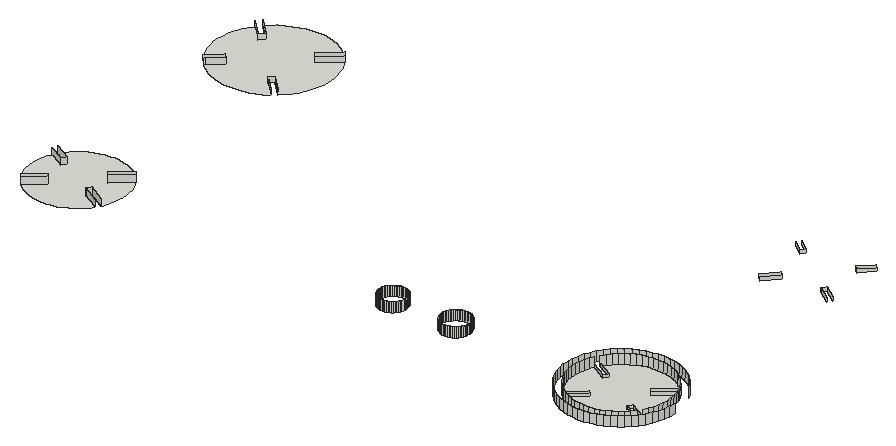
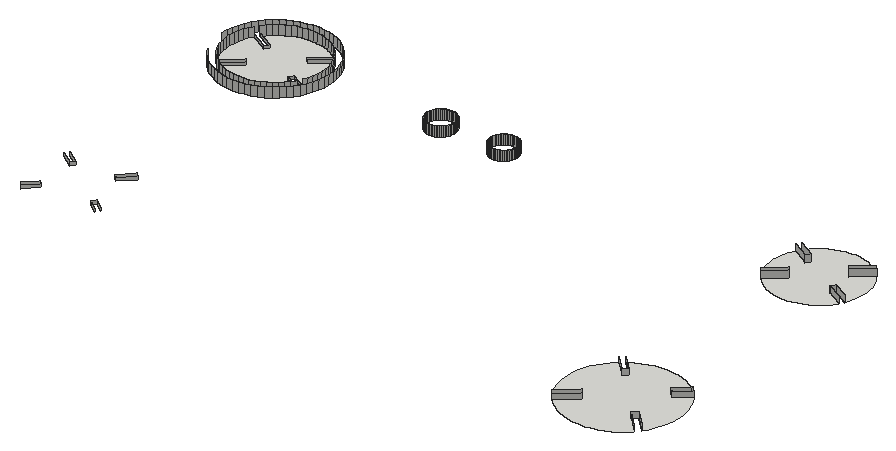
# SketchUp Ruby script. Lengths in inches.
U = 1.inch
M = Sketchup.active_model
def pt(a) = Geom::Point3d.new(a.map { |v| v * U })
def face(e, loops, mat)
  f = e.add_face(loops[0].map { |a| pt(a) })
  loops[1..].each { |l| e.add_face(l.map { |a| pt(a) }).erase! }
  f.material = f.back_material = mat if mat
  f
end
# faces: each face lists its corners as indices into pts; further lists are holes
def faces(e, pts, list, mat = nil) = list.each { |f| face(e, (f[0].is_a?(Array) ? f : [f]).map { |l| l.map { |i| pts[i] } }, mat) }
# xy, xz, yz: faces in a plane at the given z, y or x. An outline is a flat list of corners, or four numbers for a rectangle; further outlines are holes
def ring(l) = l.size == 4 ? [[l[0], l[1]], [l[2], l[1]], [l[2], l[3]], [l[0], l[3]]] : l.each_slice(2).to_a
def flat(e, list, mat, &to3) = list.each { |f| face(e, (f[0].is_a?(Array) ? f : [f]).map { |l| ring(l).map { |u, v| to3.(u, v) } }, mat) }
def xy(e, z, list, mat = nil) = flat(e, list, mat) { |x, y| [x, y, z] }
def xz(e, y, list, mat = nil) = flat(e, list, mat) { |x, z| [x, y, z] }
def yz(e, x, list, mat = nil) = flat(e, list, mat) { |y, z| [x, y, z] }
def lines(e, pts, list) = list.each { |a, b| e.add_line(pt(pts[a]), pt(pts[b])) }
# prism: a flat outline (further loops are holes) pulled along v
def prism(e, loops, v, mat = nil)
  f = face(e, loops, mat); d = Geom::Vector3d.new(v.map { |x| x * U })
  f.pushpull(f.normal.samedirection?(d) ? d.length : -d.length)
end
def box(e, o, s, mat = nil) = prism(e, [[o, [o[0] + s[0], o[1], o[2]], [o[0] + s[0], o[1] + s[1], o[2]], [o[0], o[1] + s[1], o[2]]]], [0, 0, s[2]], mat)
def at(x, y, z, deg = 0) = Geom::Transformation.translation(pt([x, y, z])) * Geom::Transformation.rotation(ORIGIN, Z_AXIS, deg.degrees)
def axes(o, x, y, z) = Geom::Transformation.new([*x, 0, *y, 0, *z, 0, *pt(o).to_a, 1])
def part(name) = M.definitions.add(name)
# library, detail: a bought-in or finely detailed component or shape, given as its bounding box
def library(name, o, s) = part(name).tap { |d| box(d.entities, o, s) }
def detail(e, o, s) = box(e.add_group.entities, o, s)
def put(e, d, t, mat = nil) = e.add_instance(d, t).tap { |i| i.material = mat if mat }
def group(e, t, mat = nil) = e.add_group.tap { |g| g.transformation = t; g.material = mat if mat }.entities
root = M.entities
xy(root,253.1875,[[844.95,632.14,846.82,632.24,848.68,632.53,850.49,633.01,852.24,633.6875,853.91,634.54,855.49,635.56,856.94,636.74,858.27,638.07,859.45,639.53,852.51,643.53,853.45,645.15,860.47,641.1,861.32,642.77,862,644.52,862.48,646.33,862.77,648.1875,862.875,650.06,862.77,651.93,862.48,653.79,862,655.6,861.32,657.35,860.47,659.02,859.45,660.59,852.77,654.76,851.61,656.05,858.27,662.05,856.94,663.38,855.49,664.56,853.91,665.58,852.24,666.43,850.49,667.1,848.68,667.59,846.82,667.88,844.95,667.98,843.08,667.88,841.23,667.59,839.41,667.1,837.66,666.43,835.99,665.58,834.42,664.56,832.96,663.38,831.63,662.05,830.45,660.59,829.43,659.02,835.82,655.33,834.88,653.71,828.58,657.35,827.91,655.6,827.42,653.79,827.13,651.93,827.03,650.06,827.13,648.1875,827.42,646.33,827.91,644.52,828.58,642.77,829.43,641.1,830.45,639.53,831.63,638.07,837.78,643.6,838.75,642.52,832.58,637.12,832.96,636.74,834.42,635.56,835.99,634.54,837.66,633.6875,839.41,633.01,841.23,632.53,843.08,632.24],[634.4375,632.64,636.26,632.71,638.07,632.96,639.84,633.41,641.55,634.04,643.19,634.84,644.73,635.81,646.16,636.93,647.47,638.2,648.64,639.6,649.15,640.36,642.53,644.09,643.42,645.67,650.09,641.92,650.51,642.73,651.19,644.42,651.69,646.17,652.01,647.97,652.13,649.79,652.0625,651.61,651.8,653.42,651.36,655.18,650.73,656.9,649.93,658.53,648.96,660.08,642.65,654.57,641.46,655.95,647.84,661.51,646.57,662.82,645.17,663.99,643.65,665.01,642.04,665.86,640.35,666.54,638.6,667.04,636.8,667.35,634.98,667.48,633.16,667.41,631.35,667.15,629.58,666.71,627.87,666.08,626.23,665.28,624.69,664.31,623.25,663.19,621.95,661.92,620.78,660.52,619.76,659,625.78,655.61,624.89,654.02,618.91,657.39,618.23,655.7,617.73,653.95,617.41,652.15,617.29,650.33,617.36,648.51,617.61,646.7,618.06,644.93,618.6875,643.22,619.49,641.58,620.46,640.04,621.58,638.6,627.88,644.1,629.08,642.73,622.85,637.29,624.25,636.125,625.77,635.11,627.38,634.26,629.07,633.58,630.82,633.08,632.62,632.76],[634.71,723.48,636.95,723.59,639.16,723.94,641.33,724.53,643.42,725.33,645.42,726.35,647.3,727.57,641.99,732.875,643.57,734.45,649.04,728.98,650.63,730.5625,652.04,732.31,653.26,734.1875,654.28,736.19,655.08,738.28,655.66,740.44,656.01,742.66,656.13,744.9,656.01,747.14,655.66,749.35,655.08,751.52,654.28,753.61,653.26,755.61,652.04,757.49,645.15,751.5625,643.67,753.28,650.63,759.23,649.04,760.82,647.3,762.23,645.42,763.45,643.42,764.47,641.33,765.27,639.16,765.85,636.95,766.2,634.71,766.32,632.47,766.2,630.26,765.85,628.09,765.27,626,764.47,624,763.45,622.12,762.23,620.375,760.82,618.79,759.23,624.74,753.28,623.16,751.71,617.38,757.49,616.16,755.61,615.14,753.61,614.34,751.52,613.76,749.35,613.41,747.14,613.29,744.9,613.41,742.66,613.76,740.44,614.34,738.28,615.14,736.19,616.16,734.1875,617.38,732.31,618.09,731.4375,623.16,735.77,624.69,733.98,619.86,729.83,619.69,729.66,620.375,728.98,622.12,727.57,624,726.35,626,725.33,628.09,724.53,630.26,723.94,632.47,723.59]])
p = [[842.78,629.42,253.1875],[844.95,629.31,253.1875],[844.95,629.31,256.875],[842.78,629.42,256.875],[847.12,629.42,253.1875],[847.12,629.42,256.875],
  [840.64,629.76,253.1875],[840.64,629.76,256.875],[849.27,629.76,253.1875],[849.27,629.76,256.875],[838.54,630.32,253.1875],[838.54,630.32,256.875],
  [851.36,630.32,253.1875],[851.36,630.32,256.875],[836.51,631.1,253.1875],[836.51,631.1,256.875],[853.39,631.1,253.1875],[853.39,631.1,256.875],
  [834.58,632.09,253.1875],[834.58,632.09,256.875],[855.33,632.09,253.1875],[855.33,632.09,256.875],[832.76,633.27,253.1875],[832.76,633.27,256.875],
  [844.95,632.14,253.1875],[843.08,632.24,253.1875],[843.08,632.24,256.875],[844.95,632.14,256.875],[846.82,632.24,253.1875],[846.82,632.24,256.875],
  [857.15,633.27,253.1875],[857.15,633.27,256.875],[841.23,632.53,253.1875],[841.23,632.53,256.875],[848.68,632.53,253.1875],[848.68,632.53,256.875],
  [839.41,633.01,253.1875],[839.41,633.01,256.875],[850.49,633.01,253.1875],[850.49,633.01,256.875],[837.66,633.6875,253.1875],[837.66,633.6875,256.875],
  [852.24,633.6875,253.1875],[852.24,633.6875,256.875],[831.07,634.64,253.1875],[831.07,634.64,256.875],[858.84,634.64,253.1875],[858.84,634.64,256.875],
  [835.99,634.54,253.1875],[835.99,634.54,256.875],[853.91,634.54,253.1875],[853.91,634.54,256.875],[834.42,635.56,253.1875],[834.42,635.56,256.875],
  [855.49,635.56,253.1875],[855.49,635.56,256.875],[829.53,636.17,253.1875],[829.53,636.17,256.875],[860.37,636.17,253.1875],[860.37,636.17,256.875],
  [832.96,636.74,253.1875],[832.96,636.74,256.875],[856.94,636.74,253.1875],[856.94,636.74,256.875],[828.16,637.86,253.1875],[828.16,637.86,256.875],
  [861.74,637.86,253.1875],[861.74,637.86,256.875],[832.58,637.12,253.1875],[832.58,637.12,254.3125],[831.63,638.07,254.3125],[831.63,638.07,256.875],
  [858.27,638.07,253.1875],[858.27,638.07,256.875],[838.75,642.52,253.1875],[838.75,642.52,254.3125],[622.85,637.29,253.1875],[629.08,642.73,253.1875],
  [629.08,642.73,255.75],[622.85,637.29,255.75],[826.98,639.68,253.1875],[826.98,639.68,256.875],[862.92,639.68,253.1875],[862.92,639.68,256.875],
  [831.63,638.07,253.1875],[830.45,639.53,253.1875],[830.45,639.53,256.875],[837.78,643.6,253.1875],[837.78,643.6,254.3125],[859.45,639.53,253.1875],
  [859.45,639.53,256.875],[859.45,639.53,254.3125],[627.88,644.1,253.1875],[621.58,638.6,253.1875],[621.58,638.6,255.75],[627.88,644.1,255.75],
  [829.43,641.1,253.1875],[829.43,641.1,256.875],[852.51,643.53,253.1875],[852.51,643.53,254.3125],[826,641.62,253.1875],[826,641.62,256.875],
  [863.91,641.62,253.1875],[863.91,641.62,256.875],[642.53,644.09,253.1875],[649.15,640.36,253.1875],[649.15,640.36,255.75],[642.53,644.09,255.75],
  [828.58,642.77,253.1875],[828.58,642.77,256.875],[860.47,641.1,253.1875],[853.45,645.15,253.1875],[853.45,645.15,254.3125],[860.47,641.1,254.3125],
  [861.32,642.77,253.1875],[860.47,641.1,256.875],[861.32,642.77,256.875],[825.22,643.65,253.1875],[825.22,643.65,256.875],[864.6875,643.65,253.1875],
  [864.6875,643.65,256.875],[650.09,641.92,253.1875],[643.42,645.67,253.1875],[643.42,645.67,255.75],[650.09,641.92,255.75],[827.91,644.52,253.1875],
  [827.91,644.52,256.875],[862,644.52,253.1875],[862,644.52,256.875],[824.66,645.74,253.1875],[824.66,645.74,256.875],[865.25,645.74,253.1875],
  [865.25,645.74,256.875],[780.65,644.47,253.1875],[781.2,644.44,253.1875],[781.2,644.44,256.875],[780.65,644.47,256.875],[781.76,644.47,253.1875],
  [781.76,644.47,256.875],[780.1,644.56,253.1875],[780.1,644.56,256.875],[782.31,644.56,253.1875],[782.31,644.56,256.875],[827.42,646.33,253.1875],
  [827.42,646.33,256.875],[862.48,646.33,253.1875],[862.48,646.33,256.875],[779.5625,644.7,253.1875],[779.5625,644.7,256.875],[782.85,644.7,253.1875],
  [782.85,644.7,256.875],[755.79,644.8,253.1875],[756.3125,644.72,253.1875],[756.3125,644.72,256.875],[755.79,644.8,256.875],[756.84,644.69,253.1875],
  [756.84,644.69,256.875],[757.37,644.72,253.1875],[757.37,644.72,256.875],[757.89,644.8,253.1875],[757.89,644.8,256.875],[779.04,644.9,253.1875],
  [779.04,644.9,256.875],[783.36,644.9,253.1875],[783.36,644.9,256.875],[755.28,644.94,253.1875],[755.28,644.94,256.875],[758.4,644.94,253.1875],
  [758.4,644.94,256.875],[754.78,645.13,253.1875],[754.78,645.13,256.875],[758.9,645.13,253.1875],[758.9,645.13,256.875],[778.55,645.15,253.1875],
  [778.55,645.15,256.875],[783.86,645.15,253.1875],[783.86,645.15,256.875],[754.31,645.37,253.1875],[754.31,645.37,256.875],[759.37,645.37,253.1875],
  [759.37,645.37,256.875],[778.08,645.46,253.1875],[778.08,645.46,256.875],[784.33,645.46,253.1875],[784.33,645.46,256.875],[753.86,645.66,253.1875],
  [753.86,645.66,256.875],[759.82,645.66,253.1875],[759.82,645.66,256.875],[777.65,645.81,253.1875],[777.65,645.81,256.875],[784.76,645.81,253.1875],
  [784.76,645.81,256.875],[753.45,645.99,253.1875],[753.45,645.99,256.875],[760.23,645.99,253.1875],[760.23,645.99,256.875],[824.32,647.89,253.1875],
  [824.32,647.89,256.875],[865.59,647.89,253.1875],[865.59,647.89,256.875],[777.26,646.2,253.1875],[777.26,646.2,256.875],[785.15,646.2,253.1875],
  [785.15,646.2,256.875],[753.08,646.37,253.1875],[753.08,646.37,256.875],[760.6,646.37,253.1875],[760.6,646.37,256.875],[776.91,646.63,253.1875],
  [776.91,646.63,256.875],[785.5,646.63,253.1875],[785.5,646.63,256.875],[827.13,648.1875,253.1875],[827.13,648.1875,256.875],[862.77,648.1875,253.1875],
  [862.77,648.1875,256.875],[752.74,646.78,253.1875],[752.74,646.78,256.875],[760.94,646.78,253.1875],[760.94,646.78,256.875],[776.6,647.1,253.1875],
  [776.6,647.1,256.875],[785.8,647.1,253.1875],[785.8,647.1,256.875],[752.46,647.22,253.1875],[752.46,647.22,256.875],[761.22,647.22,253.1875],
  [761.22,647.22,256.875],[776.35,647.59,253.1875],[776.35,647.59,256.875],[786.06,647.59,253.1875],[786.06,647.59,256.875],[752.21,647.7,253.1875],
  [752.21,647.7,256.875],[761.46,647.7,253.1875],[761.46,647.7,256.875],[776.15,648.11,253.1875],[776.15,648.11,256.875],[786.26,648.11,253.1875],
  [786.26,648.11,256.875],[752.02,648.19,253.1875],[752.02,648.19,256.875],[761.65,648.19,253.1875],[761.65,648.19,256.875],[824.2,650.06,253.1875],
  [824.2,650.06,256.875],[865.7,650.06,253.1875],[865.7,650.06,256.875],[776.01,648.65,253.1875],[776.01,648.65,256.875],[786.4,648.65,253.1875],
  [786.4,648.65,256.875],[751.89,648.7,253.1875],[751.89,648.7,256.875],[761.79,648.7,253.1875],[761.79,648.7,256.875],[827.03,650.06,253.1875],
  [827.03,650.06,256.875],[862.875,650.06,253.1875],[862.875,650.06,256.875],[775.92,649.2,253.1875],[775.92,649.2,256.875],[786.49,649.2,253.1875],
  [786.49,649.2,256.875],[751.8,649.23,253.1875],[751.8,649.23,256.875],[751.78,649.75,253.1875],[751.78,649.75,256.875],[775.89,649.75,253.1875],
  [775.89,649.75,256.875],[786.52,649.75,253.1875],[786.52,649.75,256.875],[751.8,650.28,253.1875],[751.8,650.28,256.875],[761.9,649.75,253.1875],
  [761.875,650.28,253.1875],[761.875,650.28,256.875],[761.9,649.75,256.875],[775.92,650.31,253.1875],[775.92,650.31,256.875],[786.49,650.31,253.1875],
  [786.49,650.31,256.875],[824.32,652.23,253.1875],[824.32,652.23,256.875],[827.13,651.93,253.1875],[827.13,651.93,256.875],[862.77,651.93,253.1875],
  [862.77,651.93,256.875],[751.89,650.81,253.1875],[751.89,650.81,256.875],[761.79,650.81,253.1875],[761.79,650.81,256.875],[776.01,650.86,253.1875],
  [776.01,650.86,256.875],[786.4,650.86,253.1875],[786.4,650.86,256.875],[752.02,651.32,253.1875],[752.02,651.32,256.875],[761.65,651.32,253.1875],
  [761.65,651.32,256.875],[776.15,651.4,253.1875],[776.15,651.4,256.875],[786.26,651.4,253.1875],[786.26,651.4,256.875],[752.21,651.8125,253.1875],
  [752.21,651.8125,256.875],[761.46,651.8125,253.1875],[761.46,651.8125,256.875],[776.35,651.92,253.1875],[776.35,651.92,256.875],[786.06,651.92,253.1875],
  [786.06,651.92,256.875],[752.46,652.29,253.1875],[752.46,652.29,256.875],[761.22,652.29,253.1875],[761.22,652.29,256.875],[776.6,652.41,253.1875],
  [776.6,652.41,256.875],[785.8,652.41,253.1875],[785.8,652.41,256.875],[827.42,653.79,253.1875],[827.42,653.79,256.875],[862.48,653.79,253.1875],
  [862.48,653.79,256.875],[824.66,654.375,253.1875],[824.66,654.375,256.875],[752.74,652.73,253.1875],[752.74,652.73,256.875],[760.94,652.73,253.1875],
  [760.94,652.73,256.875],[776.91,652.88,253.1875],[776.91,652.88,256.875],[785.5,652.88,253.1875],[785.5,652.88,256.875],[753.08,653.14,253.1875],
  [753.08,653.14,256.875],[760.6,653.14,253.1875],[760.6,653.14,256.875],[777.26,653.31,253.1875],[777.26,653.31,256.875],[785.15,653.31,253.1875],
  [785.15,653.31,256.875],[753.45,653.52,253.1875],[753.45,653.52,256.875],[760.23,653.52,253.1875],[760.23,653.52,256.875],[777.65,653.7,253.1875],
  [777.65,653.7,256.875],[784.76,653.7,253.1875],[784.76,653.7,256.875],[753.86,653.85,253.1875],[753.86,653.85,256.875],[759.82,653.85,253.1875],
  [759.82,653.85,256.875],[778.08,654.05,253.1875],[778.08,654.05,256.875],[784.33,654.05,253.1875],[784.33,654.05,256.875],[828.58,657.35,253.1875],
  [834.88,653.71,253.1875],[834.88,653.71,254.3125],[828.58,657.35,254.3125],[835.82,655.33,253.1875],[835.82,655.33,254.3125],[827.91,655.6,253.1875],
  [827.91,655.6,256.875],[862,655.6,253.1875],[862,655.6,256.875],[754.31,654.14,253.1875],[754.31,654.14,256.875],[759.37,654.14,253.1875],
  [759.37,654.14,256.875],[618.91,657.39,253.1875],[624.89,654.02,253.1875],[624.89,654.02,255.75],[618.91,657.39,255.75],[625.78,655.61,253.1875],
  [625.78,655.61,255.75],[754.78,654.38,253.1875],[754.78,654.38,256.875],[758.9,654.38,253.1875],[758.9,654.38,256.875],[778.55,654.36,253.1875],
  [778.55,654.36,256.875],[783.86,654.36,253.1875],[783.86,654.36,256.875],[755.28,654.57,253.1875],[755.28,654.57,256.875],[758.4,654.57,253.1875],
  [758.4,654.57,256.875],[779.04,654.61,253.1875],[779.04,654.61,256.875],[783.36,654.61,253.1875],[783.36,654.61,256.875],[825.22,656.47,253.1875],
  [825.22,656.47,256.875],[641.46,655.95,253.1875],[642.65,654.57,253.1875],[642.65,654.57,255.75],[641.46,655.95,255.75],[648.96,660.08,253.1875],
  [648.96,660.08,255.75],[755.79,654.71,253.1875],[755.79,654.71,256.875],[757.89,654.71,253.1875],[757.89,654.71,256.875],[779.5625,654.81,253.1875],
  [779.5625,654.81,256.875],[782.85,654.81,253.1875],[782.85,654.81,256.875],[756.3125,654.79,253.1875],[756.3125,654.79,256.875],[757.37,654.79,253.1875],
  [757.37,654.79,256.875],[756.84,654.82,253.1875],[756.84,654.82,256.875],[780.1,654.95,253.1875],[780.1,654.95,256.875],[782.31,654.95,253.1875],
  [782.31,654.95,256.875],[851.61,656.05,253.1875],[852.77,654.76,253.1875],[852.77,654.76,254.3125],[851.61,656.05,254.3125],[859.45,660.59,253.1875],
  [859.45,660.59,254.3125],[780.65,655.04,253.1875],[780.65,655.04,256.875],[781.2,655.07,253.1875],[781.2,655.07,256.875],[781.76,655.04,253.1875],
  [781.76,655.04,256.875],[829.43,659.02,253.1875],[829.43,659.02,254.3125],[619.76,659,253.1875],[619.76,659,255.75],[828.58,657.35,256.875],
  [861.32,657.35,253.1875],[861.32,657.35,256.875],[647.84,661.51,253.1875],[647.84,661.51,255.75],[858.27,662.05,253.1875],[858.27,662.05,254.3125],
  [826,658.5,253.1875],[826,658.5,256.875],[860.47,659.02,253.1875],[860.47,659.02,256.875],[826.98,660.43,253.1875],[826.98,660.43,256.875],
  [830.45,660.59,253.1875],[830.45,660.59,256.875],[829.43,659.02,256.875],[859.45,660.59,256.875],[828.16,662.26,253.1875],[828.16,662.26,256.875],
  [862.92,660.43,253.1875],[861.74,662.26,253.1875],[861.74,662.26,256.875],[862.92,660.43,256.875],[831.63,662.05,253.1875],[831.63,662.05,256.875],
  [832.96,663.38,253.1875],[832.96,663.38,256.875],[856.94,663.38,253.1875],[858.27,662.05,256.875],[856.94,663.38,256.875],[829.53,663.94,253.1875],
  [829.53,663.94,256.875],[860.37,663.94,253.1875],[860.37,663.94,256.875],[834.42,664.56,253.1875],[834.42,664.56,256.875],[855.49,664.56,253.1875],
  [855.49,664.56,256.875],[831.07,665.48,253.1875],[831.07,665.48,256.875],[858.84,665.48,253.1875],[858.84,665.48,256.875],[835.99,665.58,253.1875],
  [835.99,665.58,256.875],[853.91,665.58,253.1875],[853.91,665.58,256.875],[832.76,666.85,253.1875],[832.76,666.85,256.875],[857.15,666.85,253.1875],
  [857.15,666.85,256.875],[837.66,666.43,253.1875],[837.66,666.43,256.875],[852.24,666.43,253.1875],[852.24,666.43,256.875],[839.41,667.1,253.1875],
  [839.41,667.1,256.875],[850.49,667.1,253.1875],[850.49,667.1,256.875],[834.58,668.03,253.1875],[834.58,668.03,256.875],[855.33,668.03,253.1875],
  [855.33,668.03,256.875],[841.23,667.59,253.1875],[841.23,667.59,256.875],[848.68,667.59,253.1875],[848.68,667.59,256.875],[843.08,667.88,253.1875],
  [843.08,667.88,256.875],[846.82,667.88,253.1875],[846.82,667.88,256.875],[844.95,667.98,253.1875],[844.95,667.98,256.875],[836.51,669.02,253.1875],
  [836.51,669.02,256.875],[853.39,669.02,253.1875],[853.39,669.02,256.875],[838.54,669.79,253.1875],[838.54,669.79,256.875],[851.36,669.79,253.1875],
  [851.36,669.79,256.875],[840.64,670.36,253.1875],[840.64,670.36,256.875],[849.27,670.36,253.1875],[849.27,670.36,256.875],[842.78,670.7,253.1875],
  [842.78,670.7,256.875],[847.12,670.7,253.1875],[847.12,670.7,256.875],[844.95,670.81,253.1875],[844.95,670.81,256.875],[641.99,732.875,253.1875],
  [647.3,727.57,253.1875],[647.3,727.57,255.1875],[641.99,732.875,255.1875],[649.04,728.98,253.1875],[643.57,734.45,253.1875],[643.57,734.45,255.1875],
  [649.04,728.98,255.1875],[619.69,729.66,253.1875],[619.86,729.83,253.1875],[619.86,729.83,255.1875],[619.69,729.66,255.1875],[624.69,733.98,253.1875],
  [624.69,733.98,255.1875],[834.42,730.4,253.1875],[838.85,735.32,253.1875],[838.85,735.32,254.5],[834.42,730.4,254.5],[623.16,735.77,253.1875],
  [618.09,731.4375,253.1875],[618.09,731.4375,255.1875],[623.16,735.77,255.1875],[837.46,736.57,253.1875],[832.96,731.58,253.1875],[832.96,731.58,254.5],
  [837.46,736.57,254.5],[853.22,736.57,253.1875],[858.27,732.91,253.1875],[858.27,732.91,254.5],[853.22,736.57,254.5],[859.45,734.36,253.1875],
  [854.32,738.09,253.1875],[854.32,738.09,254.5],[859.45,734.36,254.5],[829.43,753.86,253.1875],[833.38,750.99,253.1875],[833.38,750.99,254.5],
  [829.43,753.86,254.5],[834.48,752.51,253.1875],[834.48,752.51,254.5],[643.67,753.28,253.1875],[645.15,751.5625,253.1875],[645.15,751.5625,255.1875],
  [643.67,753.28,255.1875],[652.04,757.49,253.1875],[652.04,757.49,255.1875],[617.38,757.49,253.1875],[623.16,751.71,253.1875],[623.16,751.71,255.1875],
  [617.38,757.49,255.1875],[624.74,753.28,253.1875],[624.74,753.28,255.1875],[830.45,755.43,253.1875],[830.45,755.43,254.5],[852.93,753.76,253.1875],
  [854.32,752.51,253.1875],[854.32,752.51,254.5],[852.93,753.76,254.5],[858.27,756.89,253.1875],[858.27,756.89,254.5],[618.79,759.23,253.1875],
  [618.79,759.23,255.1875],[650.63,759.23,253.1875],[650.63,759.23,255.1875],[856.94,758.22,253.1875],[856.94,758.22,254.5]]
faces(root,p,[[0,1,2,3],[1,4,5,2],[6,0,3,7],[4,8,9,5],[10,6,7,11],[8,12,13,9],[14,10,11,15],[12,16,17,13],
  [18,14,15,19],[16,20,21,17],[22,18,19,23],[24,25,26,27],[28,24,27,29],[20,30,31,21],[25,32,33,26],[34,28,29,35],
  [32,36,37,33],[38,34,35,39],[36,40,41,37],[42,38,39,43],[44,22,23,45],[30,46,47,31],[40,48,49,41],[50,42,43,51],
  [48,52,53,49],[54,50,51,55],[56,44,45,57],[46,58,59,47],[52,60,61,53],[62,54,55,63],[64,56,57,65],[58,66,67,59],
  [60,68,69,70,71,61],[72,62,63,73],[68,74,75,69],[76,77,78,79],[80,64,65,81],[66,82,83,67],[84,85,86,71,70],[87,84,70,88],
  [89,72,73,90,91],[92,93,94,95],[85,96,97,86],[98,89,91,99],[100,80,81,101],[82,102,103,83],[104,105,106,107],[96,108,109,97],
  [110,111,112,113],[114,110,113,115,116],[117,100,101,118],[102,119,120,103],[121,122,123,124],[74,87,88,75],[77,92,95,78],[108,125,126,109],
  [127,114,116,128],[111,98,99,112],[129,117,118,130],[119,131,132,120],[122,104,107,123],[133,134,135,136],[134,137,138,135],[139,133,136,140],
  [137,141,142,138],[125,143,144,126],[145,127,128,146],[147,139,140,148],[141,149,150,142],[151,152,153,154],[152,155,156,153],[155,157,158,156],
  [157,159,160,158],[161,147,148,162],[149,163,164,150],[165,151,154,166],[159,167,168,160],[169,165,166,170],[167,171,172,168],[173,161,162,174],
  [163,175,176,164],[177,169,170,178],[171,179,180,172],[181,173,174,182],[175,183,184,176],[185,177,178,186],[179,187,188,180],[189,181,182,190],
  [183,191,192,184],[193,185,186,194],[187,195,196,188],[197,129,130,198],[131,199,200,132],[201,189,190,202],[191,203,204,192],[205,193,194,206],
  [195,207,208,196],[209,201,202,210],[203,211,212,204],[143,213,214,144],[215,145,146,216],[217,205,206,218],[207,219,220,208],[221,209,210,222],
  [211,223,224,212],[225,217,218,226],[219,227,228,220],[229,221,222,230],[223,231,232,224],[233,225,226,234],[227,235,236,228],[237,229,230,238],
  [231,239,240,232],[241,233,234,242],[235,243,244,236],[245,197,198,246],[199,247,248,200],[249,237,238,250],[239,251,252,240],[253,241,242,254],
  [243,255,256,244],[213,257,258,214],[259,215,216,260],[261,249,250,262],[251,263,264,252],[265,253,254,266],[267,265,266,268],[269,261,262,270],
  [263,271,272,264],[273,267,268,274],[275,276,277,278],[279,269,270,280],[271,281,282,272],[283,245,246,284],[257,285,286,258],[287,259,260,288],
  [289,273,274,290],[276,291,292,277],[293,279,280,294],[281,295,296,282],[297,289,290,298],[291,299,300,292],[301,293,294,302],[295,303,304,296],
  [305,297,298,306],[299,307,308,300],[309,301,302,310],[303,311,312,304],[313,305,306,314],[307,315,316,308],[317,309,310,318],[311,319,320,312],
  [285,321,322,286],[323,287,288,324],[325,283,284,326],[327,313,314,328],[315,329,330,316],[331,317,318,332],[319,333,334,320],[335,327,328,336],
  [329,337,338,330],[339,331,332,340],[333,341,342,334],[343,335,336,344],[337,345,346,338],[347,339,340,348],[341,349,350,342],[351,343,344,352],
  [345,353,354,346],[355,347,348,356],[349,357,358,350],[359,360,361,362],[360,363,364,361],[321,365,366,322],[367,323,324,368],[369,351,352,370],
  [353,371,372,354],[373,374,375,376],[374,377,378,375],[379,369,370,380],[371,381,382,372],[383,355,356,384],[357,385,386,358],[387,379,380,388],
  [381,389,390,382],[391,383,384,392],[385,393,394,386],[395,325,326,396],[397,398,399,400],[398,401,402,399],[403,387,388,404],[389,405,406,390],
  [407,391,392,408],[393,409,410,394],[411,403,404,412],[405,413,414,406],[415,411,412,416],[413,415,416,414],[417,407,408,418],[409,419,420,410],
  [421,422,423,424],[422,425,426,423],[427,417,418,428],[429,427,428,430],[431,429,430,432],[419,431,432,420],[363,433,434,364],[377,435,436,378],
  [365,359,362,437,366],[438,367,368,439],[440,397,400,441],[442,421,424,443],[444,395,396,445],[446,438,439,447],[448,444,445,449],[433,450,451,452,434],
  [425,446,447,453,426],[454,448,449,455],[456,457,458,459],[450,460,461,451],[460,462,463,461],[464,442,443,465,466],[467,454,455,468],[457,469,470,458],
  [462,471,472,463],[473,464,466,474],[475,467,468,476],[469,477,478,470],[471,479,480,472],[481,473,474,482],[483,475,476,484],[477,485,486,478],
  [479,487,488,480],[489,481,482,490],[487,491,492,488],[493,489,490,494],[495,483,484,496],[485,497,498,486],[491,499,500,492],[501,493,494,502],
  [499,503,504,500],[505,501,502,506],[503,507,508,504],[507,505,506,508],[509,495,496,510],[497,511,512,498],[513,509,510,514],[511,515,516,512],
  [517,513,514,518],[515,519,520,516],[521,517,518,522],[519,523,524,520],[525,521,522,526],[523,525,526,524],[527,528,529,530],[531,532,533,534],
  [535,536,537,538],[536,539,540,537],[541,542,543,544],[545,546,547,548],[549,550,551,552],[532,527,530,533],[553,554,555,556],[539,545,548,540],
  [557,558,559,560],[542,549,552,543],[558,553,556,559],[561,562,563,564],[562,565,566,563],[567,568,569,570],[568,571,572,569],[573,574,575,576],
  [574,577,578,575],[565,579,580,566],[581,582,583,584],[582,585,586,583],[577,587,588,578],[589,567,570,590],[591,581,584,592]])
